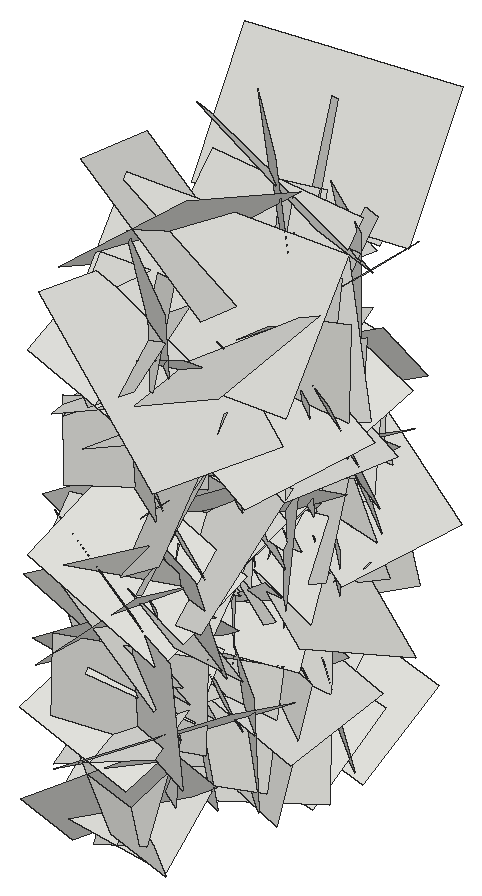
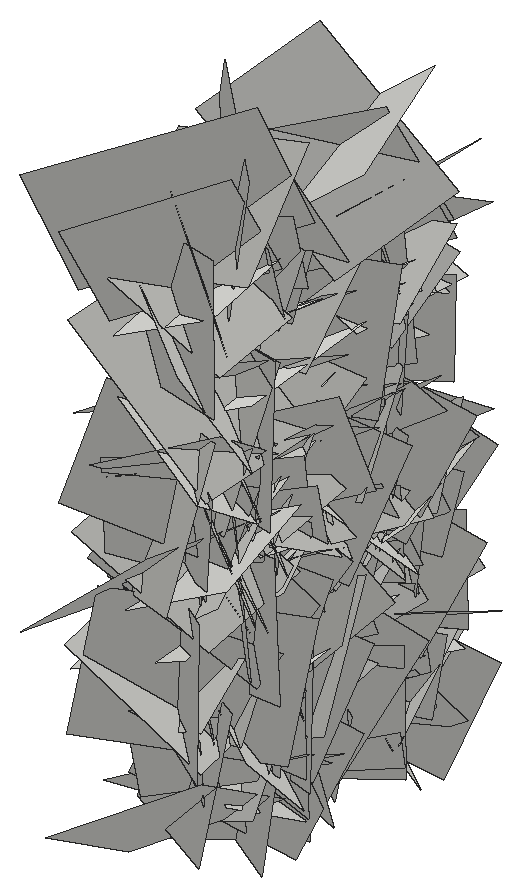
# SketchUp Ruby script. Lengths in inches.
U = 1.inch
M = Sketchup.active_model
def pt(a) = Geom::Point3d.new(a.map { |v| v * U })
def face(e, loops, mat)
  f = e.add_face(loops[0].map { |a| pt(a) })
  loops[1..].each { |l| e.add_face(l.map { |a| pt(a) }).erase! }
  f.material = f.back_material = mat if mat
  f
end
# faces: each face lists its corners as indices into pts; further lists are holes
def faces(e, pts, list, mat = nil) = list.each { |f| face(e, (f[0].is_a?(Array) ? f : [f]).map { |l| l.map { |i| pts[i] } }, mat) }
# xy, xz, yz: faces in a plane at the given z, y or x. An outline is a flat list of corners, or four numbers for a rectangle; further outlines are holes
def ring(l) = l.size == 4 ? [[l[0], l[1]], [l[2], l[1]], [l[2], l[3]], [l[0], l[3]]] : l.each_slice(2).to_a
def flat(e, list, mat, &to3) = list.each { |f| face(e, (f[0].is_a?(Array) ? f : [f]).map { |l| ring(l).map { |u, v| to3.(u, v) } }, mat) }
def xy(e, z, list, mat = nil) = flat(e, list, mat) { |x, y| [x, y, z] }
def xz(e, y, list, mat = nil) = flat(e, list, mat) { |x, z| [x, y, z] }
def yz(e, x, list, mat = nil) = flat(e, list, mat) { |y, z| [x, y, z] }
def lines(e, pts, list) = list.each { |a, b| e.add_line(pt(pts[a]), pt(pts[b])) }
# prism: a flat outline (further loops are holes) pulled along v
def prism(e, loops, v, mat = nil)
  f = face(e, loops, mat); d = Geom::Vector3d.new(v.map { |x| x * U })
  f.pushpull(f.normal.samedirection?(d) ? d.length : -d.length)
end
def box(e, o, s, mat = nil) = prism(e, [[o, [o[0] + s[0], o[1], o[2]], [o[0] + s[0], o[1] + s[1], o[2]], [o[0], o[1] + s[1], o[2]]]], [0, 0, s[2]], mat)
def at(x, y, z, deg = 0) = Geom::Transformation.translation(pt([x, y, z])) * Geom::Transformation.rotation(ORIGIN, Z_AXIS, deg.degrees)
def axes(o, x, y, z) = Geom::Transformation.new([*x, 0, *y, 0, *z, 0, *pt(o).to_a, 1])
def part(name) = M.definitions.add(name)
# library, detail: a bought-in or finely detailed component or shape, given as its bounding box
def library(name, o, s) = part(name).tap { |d| box(d.entities, o, s) }
def detail(e, o, s) = box(e.add_group.entities, o, s)
def put(e, d, t, mat = nil) = e.add_instance(d, t).tap { |i| i.material = mat if mat }
def group(e, t, mat = nil) = e.add_group.tap { |g| g.transformation = t; g.material = mat if mat }.entities
root = M.entities
c1 = part("Component\#6")
p = [[0.01,0,0],[0,3.24,4.54],[4.32,3.24,4.54],[4.33,0,0]]
faces(c1.entities,p,[[0,1,2,3]])
put(root,c1,axes([420.52,151.13,9.12],[-0.15296,0.67587,0.31221],[0.03502,0.32352,-0.68509],[0.78839,0.11676,0.09101]))
put(root,c1,axes([424.49,148.76,4.0625],[-0.10183,-0.75916,-0.2873],[-0.20096,-0.26032,0.75126],[-0.83661,0.15493,-0.14549]))
put(root,c1,axes([424.49,155.05,20.66],[-0.11898,0.43702,0.87755],[0.10329,0.88388,-0.42771],[-1.03402,0.038,-0.1437]))
put(root,c1,axes([424.49,154.79,8.7],[0.06507,0.61236,-0.89404],[0.03144,-0.89608,-0.61173],[-1.14823,0.01016,-0.06741]))
put(root,c1,axes([420.52,151.99,2.12],[-0.1775,0.68354,0.35821],[0.06031,0.37649,-0.69181],[0.81579,0.12089,0.12909]))
put(root,c1,axes([420.52,151.79,4.27],[-0.00282,-0.67031,0.14172],[-0.04158,0.14164,0.66918],[0.72504,0.00552,0.03892]))
put(root,c1,axes([420.52,147.62,1.41],[-0.08717,-0.06025,0.7019],[0.04865,0.70471,0.06586],[0.74517,-0.05306,0.07781]))
put(root,c1,axes([420.52,156.87,7.65],[0.00449,0.50233,-0.39291],[0.02578,-0.39276,-0.50188],[0.67552,0.01165,0.02176]))
put(root,c1,axes([420.52,153.92,20.8125],[0.01755,0.277,-0.54123],[0.05617,-0.54003,-0.27476],[0.64202,0.03967,0.03883]))
put(root,c1,axes([424.49,152.6,3.91],[-0.02426,0.68313,0.69515],[0.0107,0.69547,-0.68312],[-1.03305,-0.00884,-0.0234]))
put(root,c1,axes([420.52,147.13,6.96],[-0.04816,-0.19283,0.63159],[0.07038,0.62854,0.19668],[0.69645,-0.07685,0.0238]))
put(root,c1,axes([424.49,158.68,8.63],[0.07829,-0.94373,0.27717],[-0.10215,0.26967,0.94388],[-1.03759,-0.09775,-0.07202]))
put(root,c1,axes([424.49,152.91,14.99],[0.05042,0.65822,-0.8803],[0.11398,-0.87969,-0.65195],[-1.15954,-0.05785,-0.10236]))
put(root,c1,axes([424.49,159.16,9.85],[0.13765,0.1916,-1.18129],[0.14512,-1.1828,-0.17679],[-1.2602,-0.11528,-0.14939]))
put(root,c1,axes([424.49,157.06,14.03],[0.04606,-0.47436,-0.98882],[0.12961,-0.98133,0.47614],[-1.15527,-0.12901,0.01399]))
put(root,c1,axes([424.49,149.64,15.49],[0.05397,-0.71515,0.49033],[-0.26351,0.45852,0.69456],[-0.88054,-0.18105,-0.1778]))
put(root,c1,axes([420.52,148.39,13.69],[0.056,0.56116,0.2115],[0.06403,0.20626,-0.56234],[0.63244,-0.07057,0.03821]))
put(root,c1,axes([424.49,147.71,9.53],[0.0202,0.73421,-0.62443],[-0.01239,-0.62433,-0.73445],[-1.02159,0.02209,-0.00344]))
put(root,c1,axes([420.52,146.72,8.375],[0.05548,0.31048,0.67068],[-0.12303,0.66747,-0.29994],[0.77368,0.08387,-0.09579]))
put(root,c1,axes([424.49,152.28,1.18],[0.22482,-0.75958,0.923],[0.06114,0.94282,0.76264],[-1.2656,-0.08938,0.2008]))
put(root,c1,axes([424.49,154.73,4.99],[0.23466,-0.21907,1.02966],[-0.17179,1.03255,0.25453],[-1.10257,-0.20751,0.17949]))
put(root,c1,axes([420.52,148.44,10.1],[0.02371,0.59128,0.15103],[0.13632,0.14317,-0.57956],[0.63236,-0.05303,0.11928]))
put(root,c1,axes([420.52,154.81,5.31],[0.03271,-0.68931,-0.29186],[-0.0897,-0.29345,0.68411],[0.78838,-0.00479,0.08995]))
put(root,c1,axes([420.52,155.07,5.6],[-0.26442,-0.95782,0.42161],[-0.12666,0.45666,0.96674],[1.10204,-0.17733,0.21227]))
put(root,c1,axes([424.49,146.38,17.95],[-0.09245,0.38694,0.78979],[0.04684,0.79459,-0.38441],[-0.93107,0.00155,-0.09776]))
put(root,c1,axes([420.52,155.43,2.74],[0.05213,0.12024,0.7107],[-0.06472,0.71048,-0.11598],[0.7613,0.05216,-0.05853]))
put(root,c1,axes([424.49,149.03,14.67],[0.12882,0.64149,-0.81464],[-0.00451,-0.8199,-0.64626],[-1.09909,0.07855,-0.09282]))
put(root,c1,axes([420.52,145.53,10.42],[-0.22479,1.04725,-0.16356],[-0.16331,-0.19548,-1.05191],[1.11161,0.18306,-0.18761]))
put(root,c1,axes([424.49,147.21,13.43],[0.06341,1.09172,0.23851],[0.19798,0.22572,-1.08003],[-1.16785,0.09755,-0.17015]))
put(root,c1,axes([420.52,146.09,12.1875],[-0.18427,0.52878,-0.65011],[0.11203,-0.64482,-0.55274],[0.8812,0.19255,-0.06567]))
put(root,c1,axes([424.49,151.57,3.27],[-0.14157,0.02397,-0.74069],[-0.04702,-0.75154,-0.01632],[-0.78414,0.04073,0.1347]))
put(root,c1,axes([420.52,154.48,3.89],[0.11783,0.23417,0.69133],[-0.11259,0.69704,-0.21902],[0.76547,0.06648,-0.13863]))
put(root,c1,axes([420.52,152.53,7.1875],[0.08757,-0.64703,0.3684],[-0.09594,0.35919,0.65114],[0.78338,0.11632,0.03856]))
put(root,c1,axes([424.49,153.68,-0.24],[-0.08313,-0.05331,0.78078],[-0.05564,0.78328,0.04821],[-0.82769,-0.0473,-0.08166]))
put(root,c1,axes([420.52,155.23,10.47],[-0.04155,0.12694,-0.87349],[-0.11983,-0.86787,-0.12105],[0.92792,-0.10639,-0.05475]))
put(root,c1,axes([424.49,154.93,13.48],[0.13332,0.92748,-0.67904],[0.1887,-0.69057,-0.91025],[-1.20375,-0.00553,-0.2179]))
put(root,c1,axes([424.49,152.46,19.1],[0.24316,-1.11668,0.32256],[0.08367,0.34299,1.13127],[-1.22923,-0.19755,0.14081]))
put(root,c1,axes([424.49,149.625,17.57],[-0.05592,-0.7816,-0.40589],[0.0657,-0.4089,0.77935],[-0.93124,0.01809,0.07936]))
put(root,c1,axes([420.52,153.02,6.56],[0.04835,0.51462,-0.41299],[0.10228,-0.41473,-0.50612],[0.69191,0.02534,0.10368]))
put(root,c1,axes([420.52,155.74,21.65],[-0.00825,-0.17983,-0.66547],[0.14401,-0.65286,0.17483],[0.71636,0.12918,-0.04281]))
put(root,c1,axes([424.49,147.06,-0.97],[-0.01135,-0.66277,0.66685],[0.09721,0.66298,0.66039],[-0.99185,0.07256,0.05709]))
put(root,c1,axes([420.52,154.86,6.54],[-0.11481,0.21277,-0.79232],[0.09254,-0.79167,-0.22453],[0.86468,0.11298,-0.08117]))
put(root,c1,axes([424.49,155.95,10.68],[-0.04823,-0.00518,0.84226],[0.02844,0.84305,0.00663],[-0.89236,0.02715,-0.04531]))
put(root,c1,axes([424.49,146.53,12.92],[-0.03124,-0.05121,0.8385],[0.00373,0.839,0.05136],[-0.89046,0.00531,-0.0292]))
put(root,c1,axes([424.49,152.8,10.75],[0.04843,-0.82009,-0.82841],[0.32646,-0.79109,0.80013],[-1.19171,-0.25004,0.18553]))
put(root,c1,axes([420.52,155.82,10.86],[-0.10869,-0.77244,0.23734],[0.13092,0.22145,0.77409],[0.8465,-0.13343,-0.08925]))
put(root,c1,axes([420.52,156.49,11.61],[-0.16435,-0.92659,-0.48849],[-0.14398,-0.47186,0.93815],[1.10094,-0.20004,0.04977]))
put(root,c1,axes([424.49,153.88,7.81],[-0.12498,-0.19712,-0.75186],[0.05107,-0.76085,0.19192],[-0.82232,-0.01729,0.12619]))
put(root,c1,axes([420.52,154.72,7.86],[0.01434,-0.12328,-0.7123],[0.10241,-0.70572,0.12398],[0.75939,0.0975,-0.00327]))
put(root,c1,axes([424.49,155.22,14.18],[0.0107,0.67836,0.43703],[-0.08223,0.43585,-0.67474],[-0.8514,-0.03357,0.07066]))
put(root,c1,axes([420.52,152.55,8.85],[-0.17208,0.39932,0.93109],[-0.08126,0.93542,-0.41455],[1.07081,0.13515,0.11817]))
put(root,c1,axes([424.49,155.14,21.07],[0.01676,0.7943,-0.14622],[-0.08914,-0.14383,-0.79043],[-0.85145,0.03069,0.07988]))
put(root,c1,axes([420.52,158.76,13.54],[-0.17018,-0.33172,-0.9968],[-0.1229,-0.99662,0.35033],[1.10678,-0.16167,-0.11436]))
put(root,c1,axes([424.49,151.77,10.3],[-0.00621,-0.04081,-0.81439],[-0.02737,-0.814,0.04098],[-0.86391,0.02608,0.00455]))
put(root,c1,axes([424.49,149.67,1.32],[-0.10197,-0.47157,-0.58691],[0.00963,-0.59236,0.47447],[-0.798,0.05311,0.08072]))
put(root,c1,axes([420.52,154.27,5.56],[-0.10843,0.64197,-0.78685],[-0.13439,-0.79271,-0.63027],[1.06801,-0.03458,-0.15919]))
put(root,c1,axes([424.49,154.27,5.56],[0.10843,0.64197,-0.78685],[0.13439,-0.79271,-0.63027],[-1.06801,-0.03458,-0.15919]))
put(root,c1,axes([420.52,149.67,1.32],[0.10197,-0.47157,-0.58691],[-0.00963,-0.59236,0.47447],[0.798,0.05311,0.08072]))
put(root,c1,axes([420.52,151.77,10.3],[0.00621,-0.04081,-0.81439],[0.02737,-0.814,0.04098],[0.86391,0.02608,0.00455]))
put(root,c1,axes([424.49,158.76,13.54],[0.17018,-0.33172,-0.9968],[0.1229,-0.99662,0.35033],[-1.10678,-0.16167,-0.11436]))
put(root,c1,axes([420.52,155.14,21.07],[-0.01676,0.7943,-0.14622],[0.08914,-0.14383,-0.79043],[0.85145,0.03069,0.07988]))
put(root,c1,axes([424.49,152.55,8.85],[0.17208,0.39932,0.93109],[0.08126,0.93542,-0.41455],[-1.07081,0.13515,0.11817]))
put(root,c1,axes([420.52,155.22,14.18],[-0.0107,0.67836,0.43703],[0.08223,0.43585,-0.67474],[0.8514,-0.03357,0.07066]))
put(root,c1,axes([424.49,154.72,7.86],[-0.01434,-0.12328,-0.7123],[-0.10241,-0.70572,0.12398],[-0.75939,0.0975,-0.00327]))
put(root,c1,axes([420.52,153.88,7.81],[0.12498,-0.19712,-0.75186],[-0.05107,-0.76085,0.19192],[0.82232,-0.01729,0.12619]))
put(root,c1,axes([424.49,156.49,11.61],[0.16435,-0.92659,-0.48849],[0.14398,-0.47186,0.93815],[-1.10094,-0.20004,0.04977]))
put(root,c1,axes([424.49,155.82,10.86],[0.10869,-0.77244,0.23734],[-0.13092,0.22145,0.77409],[-0.8465,-0.13343,-0.08925]))
put(root,c1,axes([420.52,152.8,10.75],[-0.04843,-0.82009,-0.82841],[-0.32646,-0.79109,0.80013],[1.19171,-0.25004,0.18553]))
put(root,c1,axes([420.52,146.53,12.92],[0.03124,-0.05121,0.8385],[-0.00373,0.839,0.05136],[0.89046,0.00531,-0.0292]))
put(root,c1,axes([420.52,155.95,10.68],[0.04823,-0.00518,0.84226],[-0.02844,0.84305,0.00663],[0.89236,0.02715,-0.04531]))
put(root,c1,axes([424.49,154.86,6.54],[0.11481,0.21277,-0.79232],[-0.09254,-0.79167,-0.22453],[-0.86468,0.11298,-0.08117]))
put(root,c1,axes([420.52,147.06,-0.97],[0.01135,-0.66277,0.66685],[-0.09721,0.66298,0.66039],[0.99185,0.07256,0.05709]))
put(root,c1,axes([424.49,155.74,21.65],[0.00825,-0.17983,-0.66547],[-0.14401,-0.65286,0.17483],[-0.71636,0.12918,-0.04281]))
put(root,c1,axes([424.49,153.02,6.56],[-0.04835,0.51462,-0.41299],[-0.10228,-0.41473,-0.50612],[-0.69191,0.02534,0.10368]))
put(root,c1,axes([420.52,149.625,17.57],[0.05592,-0.7816,-0.40589],[-0.0657,-0.4089,0.77935],[0.93124,0.01809,0.07936]))
put(root,c1,axes([420.52,152.46,19.1],[-0.24316,-1.11668,0.32256],[-0.08367,0.34299,1.13127],[1.22923,-0.19755,0.14081]))
put(root,c1,axes([420.52,154.93,13.48],[-0.13332,0.92748,-0.67904],[-0.1887,-0.69057,-0.91025],[1.20375,-0.00553,-0.2179]))
put(root,c1,axes([424.49,155.23,10.47],[0.04155,0.12694,-0.87349],[0.11983,-0.86787,-0.12105],[-0.92792,-0.10639,-0.05475]))
put(root,c1,axes([420.52,153.68,-0.24],[0.08313,-0.05331,0.78078],[0.05564,0.78328,0.04821],[0.82769,-0.0473,-0.08166]))
put(root,c1,axes([424.49,152.53,7.1875],[-0.08757,-0.64703,0.3684],[0.09594,0.35919,0.65114],[-0.78338,0.11632,0.03856]))
put(root,c1,axes([424.49,154.48,3.89],[-0.11783,0.23417,0.69133],[0.11259,0.69704,-0.21902],[-0.76547,0.06648,-0.13863]))
put(root,c1,axes([420.52,151.57,3.27],[0.14157,0.02397,-0.74069],[0.04702,-0.75154,-0.01632],[0.78414,0.04073,0.1347]))
put(root,c1,axes([424.49,146.09,12.1875],[0.18427,0.52878,-0.65011],[-0.11203,-0.64482,-0.55274],[-0.8812,0.19255,-0.06567]))
put(root,c1,axes([420.52,147.21,13.43],[-0.06341,1.09172,0.23851],[-0.19798,0.22572,-1.08003],[1.16785,0.09755,-0.17015]))
put(root,c1,axes([424.49,145.53,10.42],[0.22479,1.04725,-0.16356],[0.16331,-0.19548,-1.05191],[-1.11161,0.18306,-0.18761]))
put(root,c1,axes([420.52,149.03,14.67],[-0.12882,0.64149,-0.81464],[0.00451,-0.8199,-0.64626],[1.09909,0.07855,-0.09282]))
put(root,c1,axes([424.49,155.43,2.74],[-0.05213,0.12024,0.7107],[0.06472,0.71048,-0.11598],[-0.7613,0.05216,-0.05853]))
put(root,c1,axes([420.52,146.38,17.95],[0.09245,0.38694,0.78979],[-0.04684,0.79459,-0.38441],[0.93107,0.00155,-0.09776]))
put(root,c1,axes([424.49,155.07,5.6],[0.26442,-0.95782,0.42161],[0.12666,0.45666,0.96674],[-1.10204,-0.17733,0.21227]))
put(root,c1,axes([424.49,154.81,5.31],[-0.03271,-0.68931,-0.29186],[0.0897,-0.29345,0.68411],[-0.78838,-0.00479,0.08995]))
put(root,c1,axes([424.49,148.44,10.1],[-0.02371,0.59128,0.15103],[-0.13632,0.14317,-0.57956],[-0.63236,-0.05303,0.11928]))
put(root,c1,axes([420.52,154.73,4.99],[-0.23466,-0.21907,1.02966],[0.17179,1.03255,0.25453],[1.10257,-0.20751,0.17949]))
put(root,c1,axes([420.52,152.28,1.18],[-0.22482,-0.75958,0.923],[-0.06114,0.94282,0.76264],[1.2656,-0.08938,0.2008]))
put(root,c1,axes([424.49,146.72,8.375],[-0.05548,0.31048,0.67068],[0.12303,0.66747,-0.29994],[-0.77368,0.08387,-0.09579]))
put(root,c1,axes([420.52,147.71,9.53],[-0.0202,0.73421,-0.62443],[0.01239,-0.62433,-0.73445],[1.02159,0.02209,-0.00344]))
put(root,c1,axes([424.49,148.39,13.69],[-0.056,0.56116,0.2115],[-0.06403,0.20626,-0.56234],[-0.63244,-0.07057,0.03821]))
put(root,c1,axes([420.52,149.64,15.49],[-0.05397,-0.71515,0.49033],[0.26351,0.45852,0.69456],[0.88054,-0.18105,-0.1778]))
put(root,c1,axes([420.52,157.06,14.03],[-0.04606,-0.47436,-0.98882],[-0.12961,-0.98133,0.47614],[1.15527,-0.12901,0.01399]))
put(root,c1,axes([420.52,159.16,9.85],[-0.13765,0.1916,-1.18129],[-0.14512,-1.1828,-0.17679],[1.2602,-0.11528,-0.14939]))
put(root,c1,axes([420.52,152.91,14.99],[-0.05042,0.65822,-0.8803],[-0.11398,-0.87969,-0.65195],[1.15954,-0.05785,-0.10236]))
put(root,c1,axes([420.52,158.68,8.63],[-0.07829,-0.94373,0.27717],[0.10215,0.26967,0.94388],[1.03759,-0.09775,-0.07202]))
put(root,c1,axes([424.49,147.13,6.96],[0.04816,-0.19283,0.63159],[-0.07038,0.62854,0.19668],[-0.69645,-0.07685,0.0238]))
put(root,c1,axes([420.52,152.6,3.91],[0.02426,0.68313,0.69515],[-0.0107,0.69547,-0.68312],[1.03305,-0.00884,-0.0234]))
put(root,c1,axes([424.49,153.92,20.8125],[-0.01755,0.277,-0.54123],[-0.05617,-0.54003,-0.27476],[-0.64202,0.03967,0.03883]))
put(root,c1,axes([424.49,156.87,7.65],[-0.00449,0.50233,-0.39291],[-0.02578,-0.39276,-0.50188],[-0.67552,0.01165,0.02176]))
put(root,c1,axes([424.49,147.62,1.41],[0.08717,-0.06025,0.7019],[-0.04865,0.70471,0.06586],[-0.74517,-0.05306,0.07781]))
put(root,c1,axes([424.49,151.79,4.27],[0.00282,-0.67031,0.14172],[0.04158,0.14164,0.66918],[-0.72504,0.00552,0.03892]))
put(root,c1,axes([424.49,151.99,2.12],[0.1775,0.68354,0.35821],[-0.06031,0.37649,-0.69181],[-0.81579,0.12089,0.12909]))
put(root,c1,axes([420.52,154.79,8.7],[-0.06507,0.61236,-0.89404],[-0.03144,-0.89608,-0.61173],[1.14823,0.01016,-0.06741]))
put(root,c1,axes([420.52,155.05,20.66],[0.11898,0.43702,0.87755],[-0.10329,0.88388,-0.42771],[1.03402,0.038,-0.1437]))
put(root,c1,axes([420.52,148.76,4.0625],[0.10183,-0.75916,-0.2873],[0.20096,-0.26032,0.75126],[0.83661,0.15493,-0.14549]))
put(root,c1,axes([424.49,151.13,9.12],[0.15296,0.67587,0.31221],[-0.03502,0.32352,-0.68509],[-0.78839,0.11676,0.09101]))
put(root,c1,axes([420.52,158.45,22.43],[-0.19892,0.24365,-1.12098],[0.08242,-1.13056,-0.25875],[1.21318,0.11676,-0.16622]))
put(root,c1,axes([420.52,153.47,7.93],[-0.25077,0.36385,-1.26635],[-0.08689,-1.28818,-0.35481],[1.39394,-0.01484,-0.24993]))
put(root,c1,axes([424.49,151.91,13.09],[0.06029,-0.61389,0.14039],[-0.0496,0.13645,0.61563],[-0.66568,-0.06576,-0.03315]))
put(root,c1,axes([424.49,155.37,8.05],[0.03179,-0.04018,0.69029],[0.07893,0.6871,0.03676],[-0.72868,0.07267,0.03409]))
put(root,c1,axes([424.49,147.25,18.09],[0.11506,-0.20062,0.68841],[0.02156,0.69683,0.19986],[-0.75976,-0.01061,0.10993]))
put(root,c1,axes([424.49,146,16.15],[0.10062,0.63244,0.10884],[-0.07256,0.11937,-0.63396],[-0.67636,0.08128,0.0842]))
put(root,c1,axes([420.52,157.74,11.21],[0.0595,-0.6331,0.72554],[0.06262,0.72766,0.63038],[1.01877,-0.00775,-0.08112]))
put(root,c1,axes([420.52,160.22,19.0625],[-0.13961,-0.68099,-1.03193],[-0.07146,-1.03227,0.68982],[1.30861,-0.12902,-0.07242]))
put(root,c1,axes([424.49,149.02,5.32],[0.19432,-0.67994,0.40742],[0.04988,0.42677,0.69106],[-0.83874,-0.13215,0.13549]))
put(root,c1,axes([420.52,154.9,1.8],[0.03269,0.90387,0.50014],[0.00572,0.50021,-0.90434],[1.09498,-0.0296,-0.01021]))
put(root,c1,axes([424.49,152.72,13.34],[0.14332,-0.62648,-0.12325],[-0.10799,-0.14554,0.62801],[-0.66813,-0.11086,-0.12794]))
put(root,c1,axes([420.52,157.43,12.97],[-0.1074,-0.05602,-1.35571],[-0.22854,-1.34155,0.07155],[1.42001,-0.22014,-0.09102]))
put(root,c1,axes([420.52,151.01,19.39],[0.01021,0.65154,-0.69294],[0.23408,-0.67557,-0.63214],[0.98066,0.15447,0.1581]))
put(root,c1,axes([420.52,148.31,17.26],[0.09379,0.98835,0.28145],[-0.01751,0.28383,-0.99149],[1.08916,-0.08054,-0.04018]))
put(root,c1,axes([420.52,155.4,17.52],[-0.19723,0.3027,-1.19403],[0.0763,-1.20284,-0.31615],[1.30348,0.11621,-0.16216]))
put(root,c1,axes([420.52,145.87,3.84],[0.08046,-0.07863,0.91675],[0.19442,0.90269,0.06223],[0.95574,-0.17701,-0.08983]))
put(root,c1,axes([420.52,148.09,7.11],[-0.15706,0.67864,1.02073],[0.03183,1.02986,-0.68036],[1.29889,0.05683,0.1401]))
put(root,c1,axes([420.52,148.93,-0.125],[-0.17085,0.2332,1.25619],[-0.02467,1.2654,-0.2379],[1.35409,0.05247,0.15416]))
put(root,c1,axes([420.52,158.83,13.98],[0.00743,-1.2386,0.03478],[-0.17851,0.0335,1.22715],[1.30124,0.01167,0.16814]))
put(root,c1,axes([420.52,152.08,1.74],[0.04493,0.85391,0.54577],[0.09586,0.54089,-0.85328],[1.06994,-0.08432,0.05353]))
put(root,c1,axes([420.52,151.75,19.45],[0.16935,0.44212,0.83371],[0.05466,0.84022,-0.45546],[0.99881,-0.12095,-0.11643]))
put(root,c1,axes([424.49,150.18,6.375],[0.17639,-0.58204,-0.33942],[-0.00316,-0.35025,0.59915],[-0.71419,-0.1422,-0.08648]))
put(root,c1,axes([424.49,148.65,3.04],[0.12439,-0.47488,0.46679],[0.05284,0.47892,0.47469],[-0.70386,-0.04797,0.11813]))
put(root,c1,axes([420.52,156.6875,24.44],[0.16473,0.01802,-1.18121],[-0.23771,-1.16927,-0.04735],[1.22945,-0.22849,0.14911]))
put(root,c1,axes([420.52,147.43,1.76],[0.0449,0.15818,1.07958],[0.0304,1.07985,-0.15935],[1.15617,-0.03454,-0.03773]))
put(root,c1,axes([420.52,158.38,15.93],[-0.03304,0.59909,-1.16183],[-0.1621,-1.15585,-0.5919],[1.37611,-0.12177,-0.09762]))
put(root,c1,axes([420.52,156.09,10.89],[0.02844,-1.01096,-0.23497],[0.17327,-0.228,0.99963],[1.08645,0.06282,-0.15327]))
put(root,c1,axes([420.52,159.05,4.5],[0.22831,-0.97739,-0.02602],[-0.01319,-0.02938,1.00067],[1.03632,0.21495,0.01847]))
put(root,c1,axes([420.52,157.5,5.99],[0.02733,0.34478,-1.12821],[-0.04378,-1.12752,-0.34552],[1.24973,-0.04704,0.01257]))
put(root,c1,axes([420.52,147.25,11.15],[0.01251,0.83252,-0.66438],[0.16644,-0.65852,-0.82239],[1.1167,0.08883,0.13002]))
put(root,c1,axes([420.52,153.16,13.74],[0.07693,-1.07175,0.44962],[-0.07215,0.4458,1.07364],[1.22986,0.09319,0.03486]))
put(root,c1,axes([420.52,150.33,13.2],[-0.24126,0.02501,1.36725],[0.05252,1.3853,-0.01709],[1.44858,-0.04606,0.22834]))
put(root,c1,axes([420.52,144.59,11.1],[0.20686,0.83944,0.54314],[0.00436,0.55271,-0.85571],[1.05982,-0.16612,-0.10249]))
put(root,c1,axes([420.52,153.72,24.55],[-0.10736,0.8301,-0.78481],[0.26067,-0.75358,-0.8288],[1.18252,0.24148,0.11144]))
put(root,c1,axes([420.52,148.8125,12.02],[0.02959,0.36254,-1.01381],[0.21176,-0.99828,-0.35148],[1.12146,0.17893,0.09312]))
put(root,c1,axes([420.52,148.37,14.37],[0.13394,0.02599,1.3483],[-0.3112,1.32226,0.00203],[1.39518,0.29244,-0.12899]))
put(root,c1,axes([420.52,151.84,12.71],[0.09641,-0.969,-0.91768],[-0.24854,-0.9171,0.94515],[1.39265,-0.09659,0.2322]))
put(root,c1,axes([420.52,152.41,8.09],[-0.02535,-1.06677,0.60381],[0.0625,0.60222,1.06631],[1.29785,-0.04984,-0.03955]))
put(root,c1,axes([420.52,153.41,21.56],[0.04666,0.60871,1.19242],[-0.17987,1.18598,-0.59916],[1.40769,0.13136,-0.11609]))
put(root,c1,axes([420.52,154.4,5.48],[-0.14525,-0.2612,-1.20099],[0.27145,-1.18798,0.22915],[1.27422,0.2233,-0.18571]))
put(root,c1,axes([420.52,148.05,8.79],[0.07068,0.0827,-1.14811],[0.1221,-1.14474,-0.07576],[1.21402,0.11031,0.07447]))
put(root,c1,axes([420.52,153.21,11.43],[-0.14123,-0.96535,-0.93141],[0.15435,-0.94087,0.95433],[1.41351,0.00629,-0.19727]))
put(root,c1,axes([420.52,157.09,9.16],[0.26081,-0.66319,-0.77037],[0.09697,-0.77495,0.69635],[1.07312,0.23121,0.12431]))
put(root,c1,axes([420.52,149.27,6.59],[-0.15688,1.33929,-0.00269],[0.18956,0.01708,-1.33541],[1.40693,0.14704,0.17962]))
put(root,c1,axes([420.52,149.82,11.51],[0.16938,-0.10345,1.35904],[-0.25816,1.34416,0.13095],[1.4215,0.25644,-0.13816]))
put(root,c1,axes([420.52,155.16,12.125],[0.20792,1.23942,0.0793],[-0.14973,0.10203,-1.24521],[1.30793,-0.18535,-0.15516]))
put(root,c1,axes([420.52,151.77,16.16],[0.14743,1.12249,0.38129],[0.0578,0.37744,-1.13105],[1.25528,-0.14922,0.00729]))
put(root,c1,axes([420.52,145.22,20.96],[0.20751,1.35949,-0.09859],[-0.20583,-0.07077,-1.36145],[1.43011,-0.20745,-0.18164]))
put(root,c1,axes([420.52,149.47,1.18],[0.22795,-1.08393,0.44752],[0.03192,0.45993,1.09954],[1.24263,0.18702,-0.11034]))
put(root,c1,axes([420.52,155.15,17.37],[0.02517,0.60882,-1.16754],[0.2041,-1.15679,-0.59929],[1.38075,0.1599,0.10987]))
put(root,c1,axes([420.52,146.56,18.67],[0.08115,0.67304,1.19325],[0.03541,1.19384,-0.67552],[1.45175,-0.06674,-0.05023]))
put(root,c1,axes([420.52,150.46,17.01],[0.04698,1.34267,-0.16756],[0.13374,-0.17102,-1.33703],[1.42802,-0.02815,0.13073]))
put(root,c1,axes([420.52,150.02,13.53],[0.11354,-0.10924,1.28227],[0.18202,1.27641,0.09439],[1.35193,-0.16268,-0.1204]))
put(root,c1,axes([420.52,153.54,10.59],[0.17173,1.22834,-0.55665],[0.01226,-0.5619,-1.23655],[1.42944,-0.14275,0.07748]))
put(root,c1,axes([420.52,151.36,16.73],[0.05564,-1.33407,-0.12972],[0.26745,-0.11766,1.31218],[1.39538,0.07575,-0.24633]))
put(root,c1,axes([420.52,148.21,18.05],[0.18781,1.38239,0.05917],[0.11095,0.04609,-1.39025],[1.46247,-0.18102,0.09787]))
